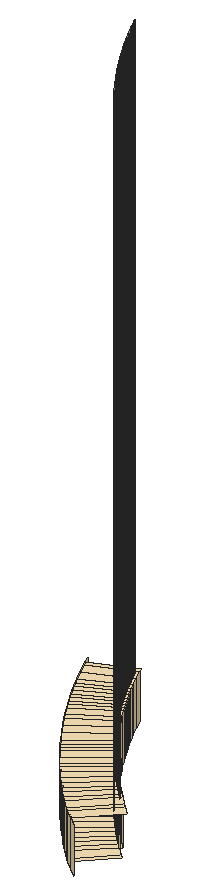
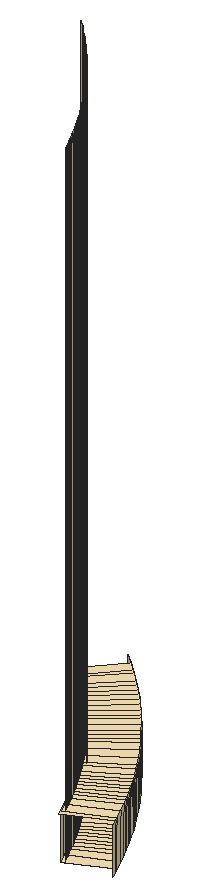
# SketchUp Ruby script. Lengths in inches.
U = 1.inch
M = Sketchup.active_model
def pt(a) = Geom::Point3d.new(a.map { |v| v * U })
def face(e, loops, mat)
  f = e.add_face(loops[0].map { |a| pt(a) })
  loops[1..].each { |l| e.add_face(l.map { |a| pt(a) }).erase! }
  f.material = f.back_material = mat if mat
  f
end
# faces: each face lists its corners as indices into pts; further lists are holes
def faces(e, pts, list, mat = nil) = list.each { |f| face(e, (f[0].is_a?(Array) ? f : [f]).map { |l| l.map { |i| pts[i] } }, mat) }
# xy, xz, yz: faces in a plane at the given z, y or x. An outline is a flat list of corners, or four numbers for a rectangle; further outlines are holes
def ring(l) = l.size == 4 ? [[l[0], l[1]], [l[2], l[1]], [l[2], l[3]], [l[0], l[3]]] : l.each_slice(2).to_a
def flat(e, list, mat, &to3) = list.each { |f| face(e, (f[0].is_a?(Array) ? f : [f]).map { |l| ring(l).map { |u, v| to3.(u, v) } }, mat) }
def xy(e, z, list, mat = nil) = flat(e, list, mat) { |x, y| [x, y, z] }
def xz(e, y, list, mat = nil) = flat(e, list, mat) { |x, z| [x, y, z] }
def yz(e, x, list, mat = nil) = flat(e, list, mat) { |y, z| [x, y, z] }
def lines(e, pts, list) = list.each { |a, b| e.add_line(pt(pts[a]), pt(pts[b])) }
# prism: a flat outline (further loops are holes) pulled along v
def prism(e, loops, v, mat = nil)
  f = face(e, loops, mat); d = Geom::Vector3d.new(v.map { |x| x * U })
  f.pushpull(f.normal.samedirection?(d) ? d.length : -d.length)
end
def box(e, o, s, mat = nil) = prism(e, [[o, [o[0] + s[0], o[1], o[2]], [o[0] + s[0], o[1] + s[1], o[2]], [o[0], o[1] + s[1], o[2]]]], [0, 0, s[2]], mat)
def at(x, y, z, deg = 0) = Geom::Transformation.translation(pt([x, y, z])) * Geom::Transformation.rotation(ORIGIN, Z_AXIS, deg.degrees)
def axes(o, x, y, z) = Geom::Transformation.new([*x, 0, *y, 0, *z, 0, *pt(o).to_a, 1])
def part(name) = M.definitions.add(name)
# library, detail: a bought-in or finely detailed component or shape, given as its bounding box
def library(name, o, s) = part(name).tap { |d| box(d.entities, o, s) }
def detail(e, o, s) = box(e.add_group.entities, o, s)
def put(e, d, t, mat = nil) = e.add_instance(d, t).tap { |i| i.material = mat if mat }
def group(e, t, mat = nil) = e.add_group.tap { |g| g.transformation = t; g.material = mat if mat }.entities
root = M.entities
M.materials.add("1026 AP 7946 SUNNY SIDE UP").color = [254, 231, 186]
xy(root,246,[[12.465,219.96,12.308,220.106,13.602,221.476,13.63,221.45,13.709,221.376,13.733,221.354,13.74,221.348],[12.308,220.106,11.925,220.474,13.239,221.822,13.261,221.802,13.366,221.7,13.378,221.688,13.389,221.678,13.448,221.622,13.537,221.537,13.554,221.52,13.571,221.505,13.602,221.476],[11.925,220.474,11.728,220.669,13.061,221.998,13.197,221.864,13.239,221.822],[11.728,220.669,11.485,220.916,12.833,222.229,12.853,222.208,12.864,222.197,13.029,222.029,13.061,221.998],[11.485,220.916,11.29,221.119,12.653,222.415,12.678,222.389,12.688,222.378,12.7,222.366,12.802,222.261,12.833,222.229],
  [11.29,221.119,11.028,221.397,12.408,222.675,12.45,222.63,12.505,222.571,12.52,222.554,12.537,222.537,12.622,222.448,12.653,222.415],[11.028,221.397,10.798,221.65,12.196,222.906,12.217,222.883,12.282,222.812,12.334,222.755,12.354,222.733,12.376,222.709,12.408,222.675],[10.798,221.65,10.519,221.964,11.935,223.199,11.954,223.178,11.997,223.129,12.027,223.095,12.06,223.058,12.117,222.994,12.165,222.941,12.19,222.913,12.196,222.906],[13.239,221.822,13.197,221.864,13.061,221.998,13.144,222.081,13.321,221.906],[10.519,221.964,10.266,222.259,11.7,223.473,11.707,223.464,11.75,223.413,11.794,223.362,11.832,223.318,11.866,223.279,11.904,223.235,11.935,223.199],
  [13.061,221.998,13.029,222.029,12.864,222.197,12.853,222.208,12.833,222.229,12.918,222.311,13.144,222.081],[12.833,222.229,12.802,222.261,12.7,222.366,12.688,222.378,12.678,222.389,12.653,222.415,12.739,222.497,12.918,222.311],[10.266,222.259,10.134,222.417,11.58,223.615,11.598,223.593,11.636,223.549,11.669,223.509,11.7,223.473],[12.653,222.415,12.622,222.448,12.537,222.537,12.52,222.554,12.505,222.571,12.45,222.63,12.408,222.675,12.495,222.756,12.739,222.497],[10.134,222.417,9.867,222.743,11.33,223.92,11.348,223.896,11.394,223.841,11.448,223.775,11.479,223.736,11.508,223.702,11.55,223.652,11.58,223.615],
  [12.408,222.675,12.376,222.709,12.354,222.733,12.334,222.755,12.282,222.812,12.217,222.883,12.196,222.906,12.285,222.987,12.495,222.756],[9.867,222.743,9.571,223.118,11.053,224.269,11.086,224.227,11.152,224.142,11.173,224.116,11.191,224.092,11.239,224.033,11.299,223.957,11.325,223.925,11.33,223.92],[12.196,222.906,12.19,222.913,12.165,222.941,12.117,222.994,12.06,223.058,12.027,223.095,11.997,223.129,11.954,223.178,11.935,223.199,12.026,223.279,12.285,222.987],[9.571,223.118,9.399,223.342,10.894,224.475,10.933,224.425,11.007,224.327,11.023,224.308,11.036,224.29,11.053,224.269],[11.935,223.199,11.904,223.235,11.866,223.279,11.832,223.318,11.794,223.362,11.75,223.413,11.707,223.464,11.7,223.473,11.792,223.551,12.026,223.279],
  [9.399,223.342,9.256,223.533,10.763,224.65,10.776,224.632,10.864,224.515,10.874,224.502,10.883,224.49,10.894,224.475],[11.7,223.473,11.669,223.509,11.636,223.549,11.598,223.593,11.58,223.615,11.674,223.693,11.792,223.551],[9.256,223.533,9.094,223.754,10.614,224.852,10.723,224.703,10.728,224.697,10.732,224.691,10.763,224.65],[11.58,223.615,11.55,223.652,11.508,223.702,11.479,223.736,11.448,223.775,11.394,223.841,11.348,223.896,11.33,223.92,11.425,223.996,11.674,223.693],[9.094,223.754,8.792,224.178,10.331,225.248,10.395,225.157,10.437,225.097,10.441,225.091,10.446,225.084,10.584,224.893,10.614,224.852],
  [11.33,223.92,11.325,223.925,11.299,223.957,11.239,224.033,11.191,224.092,11.173,224.116,11.152,224.142,11.086,224.227,11.053,224.269,11.15,224.345,11.425,223.996],[8.792,224.178,8.497,224.612,10.055,225.65,10.105,225.577,10.15,225.51,10.163,225.491,10.177,225.471,10.246,225.37,10.292,225.303,10.31,225.277,10.331,225.248],[11.053,224.269,11.036,224.29,11.023,224.308,11.007,224.327,10.933,224.425,10.894,224.475,10.993,224.55,11.15,224.345],[10.894,224.475,10.883,224.49,10.874,224.502,10.864,224.515,10.776,224.632,10.763,224.65,10.862,224.725,10.993,224.55],[8.497,224.612,8.213,225.049,9.788,226.058,9.833,225.989,9.872,225.929,9.892,225.897,9.915,225.863,9.968,225.783,10.01,225.719,10.027,225.694,10.045,225.666,10.055,225.65],
  [10.763,224.65,10.732,224.691,10.728,224.697,10.723,224.703,10.614,224.852,10.715,224.926,10.862,224.725],[10.614,224.852,10.584,224.893,10.446,225.084,10.441,225.091,10.437,225.097,10.395,225.157,10.331,225.248,10.434,225.32,10.715,224.926],[8.213,225.049,8.069,225.277,9.658,226.264,9.661,226.26,9.701,226.195,9.736,226.14,9.76,226.103,9.787,226.061,9.788,226.058],[10.331,225.248,10.31,225.277,10.292,225.303,10.246,225.37,10.177,225.471,10.163,225.491,10.15,225.51,10.105,225.577,10.055,225.65,10.161,225.721,10.434,225.32],[8.069,225.277,7.84,225.651,9.442,226.616,9.445,226.612,9.471,226.567,9.502,226.517,9.572,226.403,9.603,226.353,9.63,226.309,9.658,226.264],
  [10.055,225.65,10.045,225.666,10.027,225.694,10.01,225.719,9.968,225.783,9.915,225.863,9.892,225.897,9.872,225.929,9.833,225.989,9.788,226.058,9.897,226.127,10.161,225.721],[7.84,225.651,7.709,225.872,9.322,226.818,9.342,226.783,9.376,226.727,9.415,226.662,9.442,226.616],[7.709,225.872,7.581,226.092,9.203,227.021,9.215,227,9.251,226.938,9.294,226.864,9.32,226.822,9.322,226.818],[9.788,226.058,9.787,226.061,9.76,226.103,9.736,226.14,9.701,226.195,9.661,226.26,9.658,226.264,9.768,226.332,9.897,226.127],[7.581,226.092,7.456,226.3125,9.087,227.226,9.091,227.218,9.129,227.152,9.176,227.068,9.197,227.032,9.203,227.021],
  [9.658,226.264,9.63,226.309,9.603,226.353,9.572,226.403,9.502,226.517,9.471,226.567,9.445,226.612,9.442,226.616,9.553,226.683,9.768,226.332],[7.456,226.3125,7.346,226.512,8.984,227.41,9.008,227.367,9.06,227.273,9.076,227.245,9.087,227.226],[7.346,226.512,7.213,226.757,8.86,227.638,8.888,227.587,8.946,227.479,8.958,227.458,8.969,227.438,8.984,227.41],[9.442,226.616,9.415,226.662,9.376,226.727,9.342,226.783,9.322,226.818,9.434,226.884,9.553,226.683],[7.213,226.757,7.094,226.982,8.75,227.846,8.765,227.816,8.834,227.686,8.842,227.672,8.849,227.659,8.86,227.638],
  [9.322,226.818,9.32,226.822,9.294,226.864,9.251,226.938,9.215,227,9.203,227.021,9.317,227.086,9.434,226.884],[7.094,226.982,6.978,227.208,8.641,228.055,8.724,227.895,8.728,227.888,8.731,227.881,8.75,227.846],[9.203,227.021,9.197,227.032,9.176,227.068,9.129,227.152,9.091,227.218,9.087,227.226,9.201,227.29,9.317,227.086],[6.978,227.208,6.855,227.452,8.528,228.279,8.616,228.104,8.641,228.055],[9.087,227.226,9.076,227.245,9.06,227.273,9.008,227.367,8.984,227.41,9.1,227.473,9.201,227.29],
  [8.984,227.41,8.969,227.438,8.958,227.458,8.946,227.479,8.888,227.587,8.86,227.638,8.977,227.7,9.1,227.473],[6.855,227.452,6.642,227.892,8.329,228.688,8.357,228.628,8.392,228.554,8.399,228.541,8.406,228.526,8.471,228.395,8.503,228.329,8.506,228.322,8.51,228.315,8.528,228.279],[8.86,227.638,8.849,227.659,8.842,227.672,8.834,227.686,8.765,227.816,8.75,227.846,8.867,227.907,8.977,227.7],[8.75,227.846,8.731,227.881,8.728,227.888,8.724,227.895,8.641,228.055,8.76,228.115,8.867,227.907],[6.642,227.892,6.415,228.386,8.114,229.152,8.147,229.079,8.178,229.009,8.191,228.982,8.205,228.952,8.25,228.855,8.284,228.781,8.294,228.761,8.304,228.739,8.329,228.688],
  [8.641,228.055,8.616,228.104,8.528,228.279,8.648,228.338,8.76,228.115],[8.528,228.279,8.51,228.315,8.506,228.322,8.503,228.329,8.471,228.395,8.406,228.526,8.399,228.541,8.392,228.554,8.357,228.628,8.329,228.688,8.451,228.745,8.648,228.338],[8.329,228.688,8.304,228.739,8.294,228.761,8.284,228.781,8.25,228.855,8.205,228.952,8.191,228.982,8.178,229.009,8.147,229.079,8.114,229.152,8.238,229.208,8.451,228.745]],"1026 AP 7946 SUNNY SIDE UP")
xy(root,248,[[12.838,219.622,14.165,221.119,13.818,221.433,12.465,219.96],[12.465,219.96,13.818,221.433,13.682,221.56,12.308,220.107],[12.308,220.107,13.682,221.56,13.321,221.906,11.926,220.474],[11.926,220.474,13.321,221.906,13.144,222.081,11.728,220.669],[11.728,220.669,13.144,222.081,12.918,222.311,11.485,220.916],
  [11.485,220.916,12.918,222.311,12.739,222.497,11.29,221.119],[11.29,221.119,12.739,222.497,12.495,222.756,11.028,221.398],[11.028,221.398,12.495,222.756,12.285,222.987,10.798,221.65],[10.798,221.65,12.285,222.987,12.026,223.279,10.519,221.965],[10.519,221.965,12.026,223.279,11.793,223.551,10.266,222.259],
  [10.266,222.259,11.793,223.551,11.674,223.693,10.134,222.417],[10.134,222.417,11.674,223.693,11.425,223.996,9.867,222.743],[9.867,222.743,11.425,223.996,11.15,224.345,9.571,223.118],[9.571,223.118,11.15,224.345,10.993,224.55,9.4,223.342],[9.4,223.342,10.993,224.55,10.863,224.725,9.257,223.533],
  [9.257,223.533,10.863,224.725,10.715,224.926,9.094,223.754],[9.094,223.754,10.715,224.926,10.434,225.321,8.792,224.178],[8.792,224.178,10.434,225.321,10.162,225.721,8.497,224.612],[8.497,224.612,10.162,225.721,9.897,226.128,8.213,225.049],[8.213,225.049,9.897,226.128,9.768,226.332,8.069,225.277],
  [8.069,225.277,9.768,226.332,9.553,226.683,7.84,225.651],[7.84,225.651,9.553,226.683,9.434,226.884,7.709,225.872],[7.709,225.872,9.434,226.884,9.317,227.086,7.582,226.092],[7.582,226.092,9.317,227.086,9.201,227.29,7.457,226.3125],[7.457,226.3125,9.201,227.29,9.1,227.473,7.346,226.512],
  [7.346,226.512,9.1,227.473,8.977,227.7,7.213,226.757],[7.213,226.757,8.977,227.7,8.868,227.907,7.095,226.982],[7.095,226.982,8.868,227.907,8.76,228.115,6.978,227.208],[6.978,227.208,8.76,228.115,8.648,228.338,6.855,227.453],[6.855,227.453,8.648,228.338,8.451,228.745,6.642,227.892],
  [6.642,227.892,8.451,228.745,8.238,229.208,6.415,228.386],[6.415,228.386,8.238,229.208,8.16,229.384,6.327,228.585]],"1026 AP 7946 SUNNY SIDE UP")
p = [[13.269,219.249,246],[13.269,219.249,248],[12.838,219.622,248],[12.838,219.622,246],[12.465,219.96,248],[12.465,219.96,246],
  [12.308,220.107,248],[12.308,220.106,246],[11.926,220.474,248],[11.925,220.474,246],[11.728,220.669,248],[11.728,220.669,246],
  [11.485,220.916,248],[11.485,220.916,246],[11.29,221.119,248],[11.29,221.119,246],[11.028,221.398,248],[11.028,221.397,246],
  [10.798,221.65,248],[10.798,221.65,246],[10.519,221.965,248],[10.519,221.964,246],[13.261,221.802,246],[13.366,221.7,246],
  [13.366,221.7,274],[13.261,221.802,274],[13.208,221.853,246],[13.239,221.822,246],[13.208,221.853,274],[13.029,222.029,246],
  [13.061,221.998,246],[13.197,221.864,246],[13.197,221.864,274],[13.029,222.029,274],[13.321,221.906,248],[13.321,221.906,246],
  [13.144,222.081,246],[13.144,222.081,248],[13.203,221.858,246],[13.203,221.858,274],[10.266,222.259,248],[10.266,222.259,246],
  [12.864,222.197,246],[12.864,222.197,274],[12.918,222.311,246],[12.918,222.311,248],[12.802,222.261,246],[12.833,222.229,246],
  [12.853,222.208,246],[12.853,222.208,274],[12.802,222.261,274],[12.858,222.203,246],[12.858,222.203,274],[10.134,222.417,248],
  [10.134,222.417,246],[12.7,222.366,246],[12.7,222.366,274],[12.739,222.497,246],[12.739,222.497,248],[9.867,222.743,248],
  [9.867,222.743,246],[12.537,222.537,246],[12.622,222.448,246],[12.622,222.448,274],[12.537,222.537,274],[12.653,222.415,246],
  [12.678,222.389,246],[12.678,222.389,274],[12.688,222.378,246],[12.688,222.378,274],[12.52,222.554,246],[12.52,222.554,274],
  [12.495,222.756,246],[12.495,222.756,248],[12.376,222.709,246],[12.408,222.675,246],[12.45,222.63,246],[12.45,222.63,274],
  [12.376,222.709,274],[12.505,222.571,246],[12.505,222.571,274],[9.571,223.118,248],[9.571,223.118,246],[12.334,222.755,246],
  [12.354,222.733,246],[12.354,222.733,274],[12.334,222.755,274],[12.217,222.883,246],[12.282,222.812,246],[12.282,222.812,274],
  [12.217,222.883,274],[12.285,222.987,246],[12.285,222.987,248],[12.117,222.994,246],[12.165,222.941,246],[12.165,222.941,274],
  [12.117,222.994,274],[12.19,222.913,246],[12.19,222.913,274],[12.196,222.906,246],[12.026,223.279,246],[12.026,223.279,248],
  [12.06,223.058,246],[12.06,223.058,274],[9.4,223.342,248],[9.399,223.342,246],[11.954,223.178,246],[11.997,223.129,246],
  [11.997,223.129,274],[11.954,223.178,274],[12.027,223.095,246],[12.027,223.095,274],[11.866,223.279,246],[11.904,223.235,246],
  [11.904,223.235,274],[11.866,223.279,274],[11.935,223.199,246],[9.257,223.533,248],[9.256,223.533,246],[11.794,223.362,246],
  [11.832,223.318,246],[11.832,223.318,274],[11.794,223.362,274],[11.792,223.551,246],[11.793,223.551,248],[11.707,223.464,246],
  [11.75,223.413,246],[11.75,223.413,274],[11.707,223.464,274],[9.094,223.754,248],[9.094,223.754,246],[11.598,223.593,246],
  [11.636,223.549,246],[11.636,223.549,274],[11.598,223.593,274],[11.669,223.509,246],[11.669,223.509,274],[11.7,223.473,246],
  [11.55,223.652,246],[11.58,223.615,246],[11.55,223.652,274],[11.674,223.693,246],[11.674,223.693,248],[11.448,223.775,246],
  [11.479,223.736,246],[11.479,223.736,274],[11.448,223.775,274],[11.425,223.996,246],[11.425,223.996,248],[11.508,223.702,246],
  [11.508,223.702,274],[8.792,224.178,248],[8.792,224.178,246],[11.348,223.896,246],[11.394,223.841,246],[11.394,223.841,274],
  [11.348,223.896,274],[11.299,223.957,246],[11.325,223.925,246],[11.325,223.925,274],[11.299,223.957,274],[11.33,223.92,246],
  [11.191,224.092,246],[11.239,224.033,246],[11.239,224.033,274],[11.191,224.092,274],[11.15,224.345,246],[11.15,224.345,248],
  [11.086,224.227,246],[11.152,224.142,246],[11.152,224.142,274],[11.086,224.227,274],[11.173,224.116,246],[11.173,224.116,274],
  [8.497,224.612,248],[8.497,224.612,246],[11.036,224.29,246],[11.053,224.269,246],[11.036,224.29,274],[10.933,224.425,246],
  [11.007,224.327,246],[11.007,224.327,274],[10.933,224.425,274],[11.023,224.308,246],[11.023,224.308,274],[10.993,224.55,246],
  [10.993,224.55,248],[10.883,224.49,246],[10.894,224.475,246],[10.883,224.49,274],[10.776,224.632,246],[10.864,224.515,246],
  [10.864,224.515,274],[10.776,224.632,274],[10.874,224.502,246],[10.874,224.502,274],[10.862,224.725,246],[10.863,224.725,248],
  [8.213,225.049,248],[8.213,225.049,246],[10.732,224.691,246],[10.763,224.65,246],[10.732,224.691,274],[10.584,224.893,246],
  [10.614,224.852,246],[10.723,224.703,246],[10.723,224.703,274],[10.584,224.893,274],[10.728,224.697,246],[10.728,224.697,274],
  [10.715,224.926,246],[10.715,224.926,248],[10.446,225.084,246],[10.446,225.084,274],[10.434,225.32,246],[10.434,225.321,248],
  [8.069,225.277,248],[8.069,225.277,246],[10.395,225.157,246],[10.437,225.097,246],[10.437,225.097,274],[10.395,225.157,274],
  [10.441,225.091,246],[10.441,225.091,274],[10.31,225.277,246],[10.331,225.248,246],[10.31,225.277,274],[7.84,225.651,248],
  [7.84,225.651,246],[10.246,225.37,246],[10.292,225.303,246],[10.292,225.303,274],[10.246,225.37,274],[10.161,225.721,246],
  [10.162,225.721,248],[10.301,225.29,246],[10.301,225.29,274],[10.177,225.471,246],[10.177,225.471,274],[10.105,225.577,246],
  [10.15,225.51,246],[10.15,225.51,274],[10.105,225.577,274],[10.163,225.491,246],[10.163,225.491,274],[10.045,225.666,246],
  [10.055,225.65,246],[10.045,225.666,274],[7.709,225.872,248],[7.709,225.872,246],[9.897,226.127,246],[9.897,226.128,248],
  [9.968,225.783,246],[10.01,225.719,246],[10.01,225.719,274],[9.968,225.783,274],[10.027,225.694,246],[10.027,225.694,274],
  [9.915,225.863,246],[9.915,225.863,274],[7.582,226.092,248],[7.581,226.092,246],[9.833,225.989,246],[9.872,225.929,246],
  [9.872,225.929,274],[9.833,225.989,274],[9.892,225.897,246],[9.892,225.897,274],[9.787,226.061,246],[9.788,226.058,246],
  [9.787,226.061,274],[7.457,226.3125,248],[7.456,226.3125,246],[9.701,226.195,246],[9.736,226.14,246],[9.736,226.14,274],
  [9.701,226.195,274],[9.76,226.103,246],[9.76,226.103,274],[9.768,226.332,246],[9.768,226.332,248],[9.661,226.26,246],
  [9.661,226.26,274],[7.346,226.512,248],[7.346,226.512,246],[9.603,226.353,246],[9.63,226.309,246],[9.63,226.309,274],
  [9.603,226.353,274],[9.658,226.264,246],[9.553,226.683,246],[9.553,226.683,248],[9.537,226.46,246],[9.572,226.403,246],
  [9.572,226.403,274],[9.537,226.46,274],[7.213,226.757,248],[7.213,226.757,246],[9.471,226.567,246],[9.502,226.517,246],
  [9.502,226.517,274],[9.471,226.567,274],[9.415,226.662,246],[9.442,226.616,246],[9.445,226.612,246],[9.445,226.612,274],
  [9.415,226.662,274],[9.342,226.783,246],[9.376,226.727,246],[9.376,226.727,274],[9.342,226.783,274],[9.434,226.884,246],
  [9.434,226.884,248],[7.095,226.982,248],[7.094,226.982,246],[9.294,226.864,246],[9.32,226.822,246],[9.32,226.822,274],
  [9.294,226.864,274],[9.322,226.818,246],[9.215,227,246],[9.251,226.938,246],[9.251,226.938,274],[9.215,227,274],
  [9.317,227.086,246],[9.317,227.086,248],[6.978,227.208,248],[6.978,227.208,246],[9.176,227.068,246],[9.197,227.032,246],
  [9.197,227.032,274],[9.176,227.068,274],[9.203,227.021,246],[9.129,227.152,246],[9.129,227.152,274],[9.201,227.29,246],
  [9.201,227.29,248],[6.855,227.453,248],[6.855,227.452,246],[9.06,227.273,246],[9.076,227.245,246],[9.076,227.245,274],
  [9.06,227.273,274],[9.087,227.226,246],[9.091,227.218,246],[9.091,227.218,274],[9.008,227.367,246],[9.008,227.367,274],
  [9.1,227.473,246],[9.1,227.473,248],[8.958,227.458,246],[8.969,227.438,246],[8.969,227.438,274],[8.958,227.458,274],
  [8.984,227.41,246],[6.642,227.892,248],[6.642,227.892,246],[8.888,227.587,246],[8.946,227.479,246],[8.946,227.479,274],
  [8.888,227.587,274],[8.977,227.7,246],[8.977,227.7,248],[8.849,227.659,246],[8.86,227.638,246],[8.849,227.659,274],
  [8.765,227.816,246],[8.834,227.686,246],[8.834,227.686,274],[8.765,227.816,274],[8.842,227.672,246],[8.842,227.672,274],
  [8.867,227.907,246],[8.868,227.907,248],[8.731,227.881,246],[8.75,227.846,246],[8.731,227.881,274],[6.415,228.386,248],
  [6.415,228.386,246],[8.616,228.104,246],[8.641,228.055,246],[8.724,227.895,246],[8.724,227.895,274],[8.616,228.104,274],
  [8.728,227.888,246],[8.728,227.888,274],[8.76,228.115,246],[8.76,228.115,248],[8.51,228.315,246],[8.528,228.279,246],
  [8.51,228.315,274],[8.648,228.338,246],[8.648,228.338,248],[8.471,228.395,246],[8.503,228.329,246],[8.503,228.329,274],
  [8.471,228.395,274],[8.506,228.322,246],[8.506,228.322,274],[8.451,228.745,246],[8.451,228.745,248],[6.327,228.585,248],
  [6.327,228.585,246],[8.406,228.526,246],[8.406,228.526,274],[8.392,228.554,246],[8.399,228.541,246],[8.399,228.541,274],
  [8.392,228.554,274],[6.202,228.876,248],[6.202,228.876,246],[8.304,228.739,246],[8.329,228.688,246],[8.357,228.628,246],
  [8.357,228.628,274],[8.304,228.739,274],[8.238,229.208,246],[8.238,229.208,248],[8.294,228.761,246],[8.294,228.761,274],
  [8.25,228.855,246],[8.284,228.781,246],[8.284,228.781,274],[8.25,228.855,274],[8.205,228.952,246],[8.205,228.952,274],
  [8.178,229.009,246],[8.191,228.982,246],[8.191,228.982,274],[8.178,229.009,274]]
faces(root,p,[[0,1,2,3],[3,2,4,5],[5,4,6,7],[7,6,8,9],[9,8,10,11],[11,10,12,13],[13,12,14,15],[15,14,16,17],
  [17,16,18,19],[19,18,20,21],[22,23,24,25],[26,27,22,25,28],[29,30,31,32,33],[34,35,36,37],[31,38,39,32],[38,26,28,39],
  [21,20,40,41],[42,29,33,43],[37,36,44,45],[46,47,48,49,50],[48,51,52,49],[51,42,43,52],[41,40,53,54],[55,46,50,56],
  [45,44,57,58],[54,53,59,60],[61,62,63,64],[62,65,66,67,63],[66,68,69,67],[68,55,56,69],[70,61,64,71],[58,57,72,73],
  [74,75,76,77,78],[76,79,80,77],[79,70,71,80],[60,59,81,82],[83,84,85,86],[84,74,78,85],[87,88,89,90],[88,83,86,89],
  [73,72,91,92],[93,94,95,96],[94,97,98,95],[97,99,87,90,98],[92,91,100,101],[102,93,96,103],[82,81,104,105],[106,107,108,109],
  [107,110,111,108],[110,102,103,111],[112,113,114,115],[113,116,106,109,114],[105,104,117,118],[119,120,121,122],[120,112,115,121],[101,100,123,124],
  [125,126,127,128],[126,119,122,127],[118,117,129,130],[131,132,133,134],[132,135,136,133],[135,137,125,128,136],[138,139,131,134,140],[124,123,141,142],
  [143,144,145,146],[142,141,147,148],[144,149,150,145],[149,138,140,150],[130,129,151,152],[153,154,155,156],[154,143,146,155],[157,158,159,160],
  [158,161,153,156,159],[162,163,164,165],[163,157,160,164],[148,147,166,167],[168,169,170,171],[169,172,173,170],[172,162,165,173],[152,151,174,175],
  [176,177,168,171,178],[179,180,181,182],[180,183,184,181],[183,176,178,184],[167,166,185,186],[187,188,179,182,189],[190,191,192,193],[191,194,195,192],
  [194,187,189,195],[186,185,196,197],[175,174,198,199],[200,201,190,193,202],[203,204,205,206,207],[205,208,209,206],[208,200,202,209],[197,196,210,211],
  [212,203,207,213],[211,210,214,215],[199,198,216,217],[218,219,220,221],[219,222,223,220],[222,212,213,223],[224,225,218,221,226],[217,216,227,228],
  [229,230,231,232],[215,214,233,234],[230,235,236,231],[235,224,226,236],[237,229,232,238],[239,240,241,242],[240,243,244,241],[243,237,238,244],
  [245,246,239,242,247],[228,227,248,249],[234,233,250,251],[252,253,254,255],[253,256,257,254],[256,245,247,257],[258,252,255,259],[249,248,260,261],
  [262,263,264,265],[263,266,267,264],[266,258,259,267],[268,269,262,265,270],[261,260,271,272],[273,274,275,276],[274,277,278,275],[277,268,270,278],
  [251,250,279,280],[281,273,276,282],[272,271,283,284],[285,286,287,288],[286,289,281,282,287],[280,279,290,291],[292,293,294,295],[293,285,288,294],
  [284,283,296,297],[298,299,300,301],[299,292,295,300],[302,303,304,305,306],[304,298,301,305],[307,308,309,310],[308,302,306,309],[291,290,311,312],
  [297,296,313,314],[315,316,317,318],[316,319,307,310,317],[320,321,322,323],[321,315,318,322],[312,311,324,325],[314,313,326,327],[328,329,330,331],
  [329,332,320,323,330],[333,328,331,334],[325,324,335,336],[327,326,337,338],[339,340,341,342],[340,343,344,345,341],[344,333,334,345],[346,339,342,347],
  [336,335,348,349],[350,351,352,353],[351,354,346,347,352],[338,337,355,356],[357,358,359,360],[358,350,353,359],[349,348,361,362],[363,364,357,360,365],
  [366,367,368,369],[367,370,371,368],[370,363,365,371],[362,361,372,373],[374,375,366,369,376],[356,355,377,378],[379,380,381,382,383],[381,384,385,382],
  [384,374,376,385],[373,372,386,387],[388,389,379,383,390],[387,386,391,392],[393,394,395,396],[394,397,398,395],[397,388,390,398],[392,391,399,400],
  [378,377,401,402],[403,393,396,404],[405,406,407,408],[406,403,404,407],[402,401,409,410],[411,412,413,414,415],[413,405,408,414],[400,399,416,417],
  [418,411,415,419],[420,421,422,423],[421,418,419,422],[424,420,423,425],[426,427,428,429],[427,424,425,428]],"1026 AP 7946 SUNNY SIDE UP")
